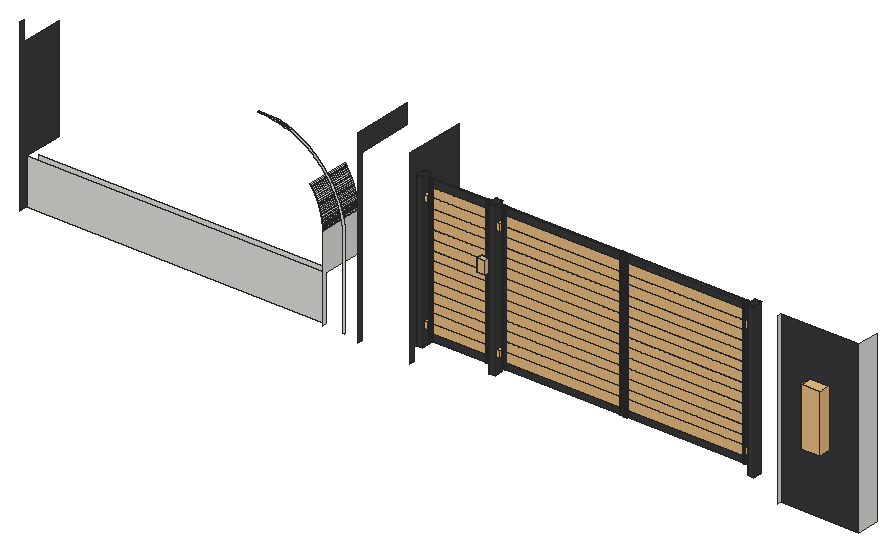
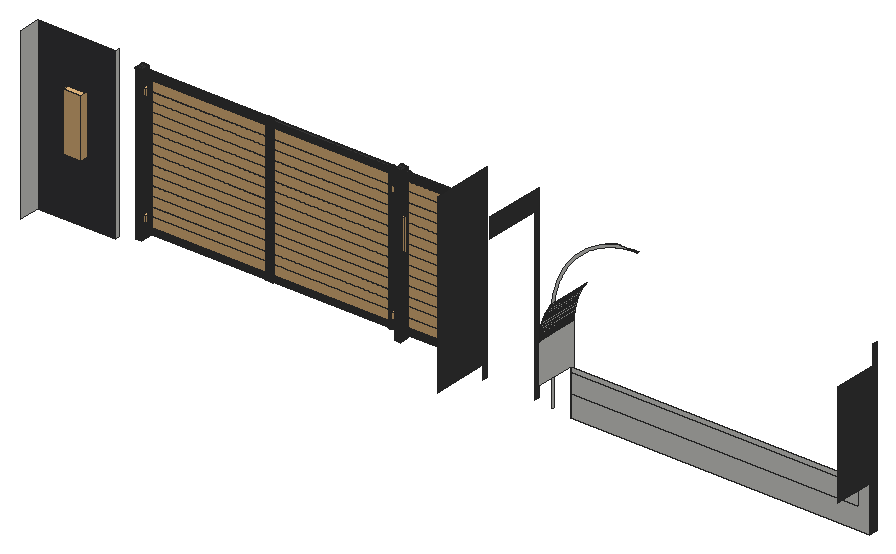
# SketchUp Ruby script. Lengths in inches.
U = 1.inch
M = Sketchup.active_model
def pt(a) = Geom::Point3d.new(a.map { |v| v * U })
def face(e, loops, mat)
  f = e.add_face(loops[0].map { |a| pt(a) })
  loops[1..].each { |l| e.add_face(l.map { |a| pt(a) }).erase! }
  f.material = f.back_material = mat if mat
  f
end
# faces: each face lists its corners as indices into pts; further lists are holes
def faces(e, pts, list, mat = nil) = list.each { |f| face(e, (f[0].is_a?(Array) ? f : [f]).map { |l| l.map { |i| pts[i] } }, mat) }
# xy, xz, yz: faces in a plane at the given z, y or x. An outline is a flat list of corners, or four numbers for a rectangle; further outlines are holes
def ring(l) = l.size == 4 ? [[l[0], l[1]], [l[2], l[1]], [l[2], l[3]], [l[0], l[3]]] : l.each_slice(2).to_a
def flat(e, list, mat, &to3) = list.each { |f| face(e, (f[0].is_a?(Array) ? f : [f]).map { |l| ring(l).map { |u, v| to3.(u, v) } }, mat) }
def xy(e, z, list, mat = nil) = flat(e, list, mat) { |x, y| [x, y, z] }
def xz(e, y, list, mat = nil) = flat(e, list, mat) { |x, z| [x, y, z] }
def yz(e, x, list, mat = nil) = flat(e, list, mat) { |y, z| [x, y, z] }
def lines(e, pts, list) = list.each { |a, b| e.add_line(pt(pts[a]), pt(pts[b])) }
# prism: a flat outline (further loops are holes) pulled along v
def prism(e, loops, v, mat = nil)
  f = face(e, loops, mat); d = Geom::Vector3d.new(v.map { |x| x * U })
  f.pushpull(f.normal.samedirection?(d) ? d.length : -d.length)
end
def box(e, o, s, mat = nil) = prism(e, [[o, [o[0] + s[0], o[1], o[2]], [o[0] + s[0], o[1] + s[1], o[2]], [o[0], o[1] + s[1], o[2]]]], [0, 0, s[2]], mat)
def at(x, y, z, deg = 0) = Geom::Transformation.translation(pt([x, y, z])) * Geom::Transformation.rotation(ORIGIN, Z_AXIS, deg.degrees)
def axes(o, x, y, z) = Geom::Transformation.new([*x, 0, *y, 0, *z, 0, *pt(o).to_a, 1])
def part(name) = M.definitions.add(name)
# library, detail: a bought-in or finely detailed component or shape, given as its bounding box
def library(name, o, s) = part(name).tap { |d| box(d.entities, o, s) }
def detail(e, o, s) = box(e.add_group.entities, o, s)
def put(e, d, t, mat = nil) = e.add_instance(d, t).tap { |i| i.material = mat if mat }
def group(e, t, mat = nil) = e.add_group.tap { |g| g.transformation = t; g.material = mat if mat }.entities
root = M.entities
M.materials.add("1432 AP 8245 TAR ROAD").color = [57, 57, 60]
M.materials.add("[Color M06]").color = [58, 58, 58]
M.materials.add("[Granite Dark Gray]").color = [61, 60, 60]
c1 = library("WALL LIGHT 61",[-1.86,-2.6875,-10.98],[8.43,8.43,26.69])
c2 = part("lamel up")
xy(c2.entities,0,[[[41.063,0.29,42.441,2.047],[41.122,0.389,42.343,1.973]],[[3.268,0.315,4.646,2.047],[3.327,0.389,4.587,1.973]]])
xy(c2.entities,4.331,[[3.327,0.439,4.587,1.924],[41.122,0.439,42.343,1.924]])
xy(c2.entities,4.724,[[4.646,0.439,41.063,1.924]])
xy(c2.entities,7.874,[[[3.268,0.315,4.646,0.315,4.646,0.439,41.063,0.439,41.063,0.315,42.441,0.315,42.441,2.047,41.063,2.047,41.063,1.924,4.646,1.924,4.646,2.047,3.268,2.047],[3.327,0.389,3.327,1.973,4.587,1.973,4.587,1.924,3.327,1.924,3.327,0.439,4.587,0.439,4.587,0.389],[41.122,0.389,41.122,0.439,42.343,0.439,42.343,1.924,41.122,1.924,41.122,1.973,42.343,1.973,42.343,0.389]]])
xz(c2.entities,0.315,[[3.268,0,4.646,7.874]])
xz(c2.entities,0.389,[[3.327,0,4.587,7.874],[41.122,0,42.343,7.874]])
xz(c2.entities,0.439,[[3.327,4.331,4.587,7.874],[41.122,4.331,42.343,7.874],[4.646,4.724,41.063,7.874]])
xz(c2.entities,1.924,[[3.327,4.331,4.587,7.874],[41.122,4.331,42.343,7.874],[4.646,4.724,41.063,7.874]])
xz(c2.entities,1.973,[[3.327,0,4.587,7.874],[41.122,0,42.343,7.874]])
xz(c2.entities,2.047,[[3.268,0,4.646,7.874],[41.063,0,42.441,7.874]])
yz(c2.entities,3.268,[[0.315,0,2.047,7.874]])
yz(c2.entities,3.327,[[0.389,0,1.973,0,1.973,7.874,1.924,7.874,1.924,4.331,0.439,4.331,0.439,7.874,0.389,7.874],[0.439,4.331,1.924,7.874]])
yz(c2.entities,4.587,[[0.389,0,0.389,7.874,0.439,7.874,0.439,4.331,0.394,0],[0.394,0,0.439,4.331,1.924,4.331,1.969,0],[1.969,0,1.924,4.331,1.924,7.874,1.973,7.874,1.973,0]])
yz(c2.entities,4.646,[[0.315,0,2.047,0,2.047,7.874,1.924,7.874,1.924,4.724,0.439,4.724,0.439,7.874,0.315,7.874]])
yz(c2.entities,41.063,[[0.29,0,0.315,7.874,0.439,7.874,0.439,4.724,1.924,4.724,1.924,7.874,2.047,7.874,2.047,0]])
yz(c2.entities,41.122,[[0.389,0,0.394,0,0.389,2.887,0.439,4.331,0.439,7.874,0.389,7.874],[0.394,0,1.969,0,1.973,2.943,1.924,4.331,0.439,4.331,0.389,2.887],[1.969,0,1.973,0,1.973,7.874,1.924,7.874,1.924,4.331,1.973,2.943]])
yz(c2.entities,42.343,[[0.389,0,0.389,7.874,0.439,7.874,0.439,4.331,1.924,4.331,1.924,7.874,1.973,7.874,1.973,0],[0.439,4.331,1.924,7.874]])
yz(c2.entities,42.441,[[0.29,0,2.047,0,2.047,7.874,0.315,7.874]])
p = [[42.441,0.29,0],[42.441,0.315,7.874],[41.063,0.315,7.874],[41.063,0.29,0]]
faces(c2.entities,p,[[0,1,2,3]])
c3 = library("lamel",[3.23,0.1,0.39],[36.57,1.38,4.33])
c4 = part("Gate stile")
xy(c4.entities,0,[[0.08,0.39,0.16,0.47],[0.16,0.39,0.16,0.47,1.57,0.47,1.57,0.59,1.65,0.59,1.65,0.39],[1.65,0.39,1.65,0.59,1.71,0.59,1.71,0.45,2.52,0.45,2.52,0.39],[0.08,0.47,0.08,1.97,1.65,1.97,1.65,1.77,1.57,1.77,1.57,1.89,0.16,1.89,0.16,0.47],[1.65,1.77,1.65,1.97,2.52,1.97,2.52,1.91,1.71,1.91,1.71,1.77]])
xy(c4.entities,3.15,[[1.57,0.59,1.65,1.77],[1.65,0.59,1.71,1.77]])
xy(c4.entities,63.78,[[1.57,0.59,1.65,1.77],[1.65,0.59,1.71,1.77]])
xy(c4.entities,66.93,[[0.08,0.39,1.65,0.39,1.65,0.59,1.57,0.59,1.57,0.47,0.16,0.47,0.16,1.89,1.57,1.89,1.57,1.77,1.65,1.77,1.65,1.97,0.08,1.97],[1.65,0.39,2.52,0.39,2.52,0.45,1.71,0.45,1.71,0.59,1.65,0.59],[1.65,1.77,1.71,1.77,1.71,1.91,2.52,1.91,2.52,1.97,1.65,1.97]])
xz(c4.entities,0.39,[[0.08,0,1.65,66.93],[1.65,0,2.52,66.93]])
xz(c4.entities,0.45,[[1.71,0,2.52,66.93]])
xz(c4.entities,0.47,[[0.16,0,1.57,66.93]])
xz(c4.entities,0.59,[[1.57,0,1.65,3.15],[1.65,0,1.71,3.15],[1.57,63.78,1.65,66.93],[1.65,63.78,1.71,66.93]])
xz(c4.entities,1.77,[[1.57,0,1.65,3.15],[1.65,0,1.71,3.15],[1.57,63.78,1.65,66.93],[1.65,63.78,1.71,66.93]])
xz(c4.entities,1.89,[[0.16,0,1.57,66.93]])
xz(c4.entities,1.91,[[1.71,0,2.52,66.93]])
xz(c4.entities,1.97,[[0.08,0,1.65,66.93],[1.65,0,2.52,66.93]])
yz(c4.entities,0.08,[[0.39,0,1.97,66.93]])
yz(c4.entities,0.16,[[0.47,0,1.89,66.93]])
yz(c4.entities,1.57,[[0.47,0,0.59,3.15],[1.77,0,1.89,3.15],[0.47,3.15,0.59,63.78],[0.59,3.15,0.59,63.78,1.77,3.15],[1.77,3.15,0.59,63.78,1.76,9.24],
  [1.77,3.15,1.76,9.24,1.89,3.15],[1.89,3.15,1.76,9.24,1.77,63.78,1.89,63.78],[1.76,9.24,0.59,63.78,1.77,63.78],[0.47,63.78,0.59,66.93],[1.77,63.78,1.89,66.93]])
yz(c4.entities,1.65,[[0.39,0,0.59,0,0.59,3.15,1.77,3.15,1.77,0,1.97,0,1.97,66.93,1.77,66.93,1.77,63.78,0.59,63.78,0.59,66.93,0.39,66.93]])
yz(c4.entities,1.71,[[0.45,0,0.59,0,0.59,3.15,1.77,3.15,1.77,0,1.91,0,1.91,63.78,0.45,63.78],[0.45,63.78,0.59,66.93],[1.77,63.78,1.91,66.93]])
yz(c4.entities,2.52,[[0.39,0,0.45,66.93],[1.91,0,1.97,66.93]])
c5 = part("Gate post")
xy(c5.entities,-3.9375,[[0.2,0.2,4.13,4.13]])
xy(c5.entities,66.93,[[[0,0,4.33,4.33],[0.2,0.2,4.13,4.13]]])
xy(c5.entities,67.01,[[0.2,0.2,4.13,4.13]])
xy(c5.entities,67.52,[[1.3,1.3,3.03,3.03]])
xz(c5.entities,0,[[0,66.93,4.33,67.01]])
xz(c5.entities,0.2,[[0.2,-3.9375,4.13,66.93],[0.2,66.93,4.13,67.01]])
xz(c5.entities,4.13,[[0.2,-3.9375,4.13,66.93],[0.2,66.93,4.13,67.01]])
xz(c5.entities,4.33,[[0,66.93,4.33,67.01]])
yz(c5.entities,0,[[0,66.93,4.33,67.01]])
yz(c5.entities,0.2,[[0.2,-3.9375,4.13,66.93],[0.2,66.93,4.13,67.01]])
yz(c5.entities,4.13,[[0.2,-3.9375,4.13,66.93],[0.2,66.93,4.13,67.01]])
yz(c5.entities,4.33,[[0,66.93,4.33,67.01]])
p = [[1.3,1.3,67.52],[1.3,3.03,67.52],[0,4.33,67.01],[0,0,67.01],[4.33,0,67.01],[3.03,1.3,67.52],
  [4.33,4.33,67.01],[3.03,3.03,67.52]]
faces(c5.entities,p,[[0,1,2,3],[4,5,0,3],[4,6,7,5],[2,1,7,6]])
c6 = library("skp6A9D",[-1.57,-1.57,-0.47],[3.14,3.14,2.95])
c7 = library("skp798A",[-3.31,-3.5,-20.01],[6.62,4.76,40.02])
c8 = library("Handle",[560.53,1368.21,-900.68],[5,2.66,5.75])
c9 = library("lamel\#1",[-36.14,0.1,0.39],[75.94,1.38,4.33])
c10 = part("lamel up\#1")
xy(c10.entities,0,[[[41.063,0.29,42.441,2.047],[41.122,0.389,42.343,1.973]],[[-36.102,0.315,-34.724,2.047],[-36.043,0.389,-34.783,1.973]]])
xy(c10.entities,4.331,[[-36.043,0.439,-34.783,1.924],[41.122,0.439,42.343,1.924]])
xy(c10.entities,4.724,[[-34.724,0.439,41.063,1.924]])
xy(c10.entities,7.874,[[[-36.102,0.315,-34.724,0.315,-34.724,0.439,41.063,0.439,41.063,0.315,42.441,0.315,42.441,2.047,41.063,2.047,41.063,1.924,-34.724,1.924,-34.724,2.047,-36.102,2.047],[-36.043,0.389,-36.043,1.973,-34.783,1.973,-34.783,1.924,-36.043,1.924,-36.043,0.439,-34.783,0.439,-34.783,0.389],[41.122,0.389,41.122,0.439,42.343,0.439,42.343,1.924,41.122,1.924,41.122,1.973,42.343,1.973,42.343,0.389]]])
xz(c10.entities,0.315,[[-36.102,0,-34.724,7.874]])
xz(c10.entities,0.389,[[-36.043,0,-34.783,7.874],[41.122,0,42.343,7.874]])
xz(c10.entities,0.439,[[-36.043,4.331,-34.783,7.874],[41.122,4.331,42.343,7.874],[-34.724,4.724,41.063,7.874]])
xz(c10.entities,1.924,[[-36.043,4.331,-34.783,7.874],[41.122,4.331,42.343,7.874],[-34.724,4.724,41.063,7.874]])
xz(c10.entities,1.973,[[-36.043,0,-34.783,7.874],[41.122,0,42.343,7.874]])
xz(c10.entities,2.047,[[-36.102,0,-34.724,7.874],[41.063,0,42.441,7.874]])
yz(c10.entities,-36.102,[[0.315,0,2.047,7.874]])
yz(c10.entities,-36.043,[[0.389,0,1.973,0,1.973,7.874,1.924,7.874,1.924,4.331,0.439,4.331,0.439,7.874,0.389,7.874],[0.439,4.331,1.924,7.874]])
yz(c10.entities,-34.783,[[0.389,0,0.389,7.874,0.439,7.874,0.439,4.331,0.394,0],[0.394,0,0.439,4.331,1.924,4.331,1.969,0],[1.969,0,1.924,4.331,1.924,7.874,1.973,7.874,1.973,0]])
yz(c10.entities,-34.724,[[0.315,0,2.047,0,2.047,7.874,1.924,7.874,1.924,4.724,0.439,4.724,0.439,7.874,0.315,7.874]])
yz(c10.entities,41.063,[[0.29,0,0.315,7.874,0.439,7.874,0.439,4.724,1.924,4.724,1.924,7.874,2.047,7.874,2.047,0]])
yz(c10.entities,41.122,[[0.389,0,0.394,0,0.389,2.887,0.439,4.331,0.439,7.874,0.389,7.874],[0.394,0,1.969,0,1.973,2.943,1.924,4.331,0.439,4.331,0.389,2.887],[1.969,0,1.973,0,1.973,7.874,1.924,7.874,1.924,4.331,1.973,2.943]])
yz(c10.entities,42.343,[[0.389,0,0.389,7.874,0.439,7.874,0.439,4.331,1.924,4.331,1.924,7.874,1.973,7.874,1.973,0],[0.439,4.331,1.924,7.874]])
yz(c10.entities,42.441,[[0.29,0,2.047,0,2.047,7.874,0.315,7.874]])
p = [[42.441,0.29,0],[42.441,0.315,7.874],[41.063,0.315,7.874],[41.063,0.29,0]]
faces(c10.entities,p,[[0,1,2,3]])
c11 = part("lamel up\#2")
xy(c11.entities,0,[[[41.063,0.29,42.441,2.047],[41.122,0.389,42.343,1.973]],[[-36.102,0.315,-34.724,2.047],[-36.043,0.389,-34.783,1.973]]])
xy(c11.entities,4.331,[[-36.043,0.439,-34.783,1.924],[41.122,0.439,42.343,1.924]])
xy(c11.entities,4.724,[[-34.724,0.439,41.063,1.924]])
xy(c11.entities,7.874,[[[-36.102,0.315,-34.724,0.315,-34.724,0.439,41.063,0.439,41.063,0.315,42.441,0.315,42.441,2.047,41.063,2.047,41.063,1.924,-34.724,1.924,-34.724,2.047,-36.102,2.047],[-36.043,0.389,-36.043,1.973,-34.783,1.973,-34.783,1.924,-36.043,1.924,-36.043,0.439,-34.783,0.439,-34.783,0.389],[41.122,0.389,41.122,0.439,42.343,0.439,42.343,1.924,41.122,1.924,41.122,1.973,42.343,1.973,42.343,0.389]]])
xz(c11.entities,0.315,[[-36.102,0,-34.724,7.874]])
xz(c11.entities,0.389,[[-36.043,0,-34.783,7.874],[41.122,0,42.343,7.874]])
xz(c11.entities,0.439,[[-36.043,4.331,-34.783,7.874],[41.122,4.331,42.343,7.874],[-34.724,4.724,41.063,7.874]])
xz(c11.entities,1.924,[[-36.043,4.331,-34.783,7.874],[41.122,4.331,42.343,7.874],[-34.724,4.724,41.063,7.874]])
xz(c11.entities,1.973,[[-36.043,0,-34.783,7.874],[41.122,0,42.343,7.874]])
xz(c11.entities,2.047,[[-36.102,0,-34.724,7.874],[41.063,0,42.441,7.874]])
yz(c11.entities,-36.102,[[0.315,0,2.047,7.874]])
yz(c11.entities,-36.043,[[0.389,0,1.973,0,1.973,7.874,1.924,7.874,1.924,4.331,0.439,4.331,0.439,7.874,0.389,7.874],[0.439,4.331,1.924,7.874]])
yz(c11.entities,-34.783,[[0.389,0,0.389,7.874,0.439,7.874,0.439,4.331,0.394,0],[0.394,0,0.439,4.331,1.924,4.331,1.969,0],[1.969,0,1.924,4.331,1.924,7.874,1.973,7.874,1.973,0]])
yz(c11.entities,-34.724,[[0.315,0,2.047,0,2.047,7.874,1.924,7.874,1.924,4.724,0.439,4.724,0.439,7.874,0.315,7.874]])
yz(c11.entities,41.063,[[0.29,0,0.315,7.874,0.439,7.874,0.439,4.724,1.924,4.724,1.924,7.874,2.047,7.874,2.047,0]])
yz(c11.entities,41.122,[[0.389,0,0.394,0,0.389,2.887,0.439,4.331,0.439,7.874,0.389,7.874],[0.394,0,1.969,0,1.973,2.943,1.924,4.331,0.439,4.331,0.389,2.887],[1.969,0,1.973,0,1.973,7.874,1.924,7.874,1.924,4.331,1.973,2.943]])
yz(c11.entities,42.343,[[0.389,0,0.389,7.874,0.439,7.874,0.439,4.331,1.924,4.331,1.924,7.874,1.973,7.874,1.973,0],[0.439,4.331,1.924,7.874]])
yz(c11.entities,42.441,[[0.29,0,2.047,0,2.047,7.874,0.315,7.874]])
p = [[42.441,0.29,0],[42.441,0.315,7.874],[41.063,0.315,7.874],[41.063,0.29,0]]
faces(c11.entities,p,[[0,1,2,3]])
c12 = part("170_fin_black_gate")
put(c12.entities,c2,axes([44.17,-0.15,7.875],[-1,0,0],[0,0.79545,0],[0,0,-1]),"[Color M06]")
put(c12.entities,c3,at(42.85,1.57,41.73,-180),"[Color M06]")
put(c12.entities,c3,at(42.85,1.57,28.74,-180),"[Color M06]")
put(c12.entities,c3,at(42.85,1.57,54.72,-180),"[Color M06]")
put(c12.entities,c3,at(42.85,1.57,37.4,-180),"[Color M06]")
put(c12.entities,c3,at(42.85,1.57,46.0625,-180),"[Color M06]")
put(c12.entities,c3,at(42.85,1.57,50.39,-180),"[Color M06]")
put(c12.entities,c3,at(42.85,1.57,20.08,-180),"[Color M06]")
put(c12.entities,c3,at(42.85,1.57,7.09,-180),"[Color M06]")
put(c12.entities,c4,at(1.56,-0.39,0),"[Color M06]")
put(c12.entities,c2,axes([44.17,1.73,59.06],[-1,0,0],[0,-0.79545,0],[0,0,1]),"[Color M06]")
put(c12.entities,c3,at(42.85,1.57,24.41,-180),"[Color M06]")
put(c12.entities,c3,at(42.85,1.57,33.07,-180),"[Color M06]")
put(c12.entities,c3,at(42.85,1.57,15.75,-180),"[Color M06]")
put(c12.entities,c3,at(42.85,1.57,11.42,-180),"[Color M06]")
put(c12.entities,c3,at(42.85,1.57,2.76,-180),"[Color M06]")
put(c12.entities,c4,at(41.08,1.97,0,-180),"[Color M06]")
put(c12.entities,c3,at(42.85,1.57,59.06,-180),"[Color M06]")
put(c12.entities,c5,at(41.94,-1.42,0.59),"[Color M06]")
put(c12.entities,c5,at(-4.89,-1.42,0.59),"[Color M06]")
put(c12.entities,c6,axes([-0.76,0.79,58.55],[0,0.9966,0],[0,0,0.9966],[0.9966,0,0]),"[Color M06]")
put(c12.entities,c6,axes([-0.76,0.79,6.11],[0,0.9966,0],[0,0,0.9966],[0.9966,0,0]),"[Color M06]")
put(c12.entities,c7,axes([41.58,1.03,41.4],[0,-0.3825,0],[0.4425,0,0],[0,0,0.36105]),"[Color M06]")
put(c12.entities,c8,axes([601.55,-1370.97,938.8125],[-1,0,0],[0,1,0],[0,0,1]),"[Color M06]")
put(c12.entities,c9,at(89.77,1.67,33.07,-180),"[Color M06]")
put(c12.entities,c10,axes([91.09,1.82,59.06],[-1,0,0],[0,-0.79545,0],[0,0,1]),"[Color M06]")
put(c12.entities,c9,at(89.77,1.67,37.4,-180),"[Color M06]")
put(c12.entities,c9,at(89.77,1.67,41.73,-180),"[Color M06]")
put(c12.entities,c9,at(89.77,1.67,59.06,-180),"[Color M06]")
put(c12.entities,c4,at(127.37,2.0625,0,-180),"[Color M06]")
put(c12.entities,c9,at(89.77,1.67,46.0625,-180),"[Color M06]")
put(c12.entities,c9,at(89.77,1.67,54.72,-180),"[Color M06]")
put(c12.entities,c9,at(89.77,1.67,50.39,-180),"[Color M06]")
put(c12.entities,c9,at(89.77,1.67,7.09,-180),"[Color M06]")
put(c12.entities,c9,at(89.77,1.67,11.42,-180),"[Color M06]")
put(c12.entities,c9,at(89.77,1.67,28.74,-180),"[Color M06]")
put(c12.entities,c11,axes([91.09,-0.06,7.875],[-1,0,0],[0,0.79545,0],[0,0,-1]),"[Color M06]")
put(c12.entities,c4,at(48.47,-0.3,0),"[Color M06]")
put(c12.entities,c9,at(89.77,1.67,15.75,-180),"[Color M06]")
put(c12.entities,c9,at(89.77,1.67,24.41,-180),"[Color M06]")
put(c12.entities,c9,at(89.77,1.67,2.76,-180),"[Color M06]")
put(c12.entities,c9,at(89.77,1.67,20.08,-180),"[Color M06]")
put(c12.entities,c9,at(168.98,1.67,15.75,-180),"[Color M06]")
put(c12.entities,c9,at(168.98,1.67,24.41,-180),"[Color M06]")
put(c12.entities,c9,at(168.98,1.67,50.39,-180),"[Color M06]")
put(c12.entities,c4,at(127.68,-0.3,0),"[Color M06]")
put(c12.entities,c9,at(168.98,1.67,46.0625,-180),"[Color M06]")
put(c12.entities,c11,axes([170.3,-0.06,7.875],[-1,0,0],[0,0.79545,0],[0,0,-1]),"[Color M06]")
put(c12.entities,c9,at(168.98,1.67,2.76,-180),"[Color M06]")
put(c12.entities,c9,at(168.98,1.67,54.72,-180),"[Color M06]")
put(c12.entities,c9,at(168.98,1.67,11.42,-180),"[Color M06]")
put(c12.entities,c9,at(168.98,1.67,7.09,-180),"[Color M06]")
put(c12.entities,c9,at(168.98,1.67,28.74,-180),"[Color M06]")
put(c12.entities,c9,at(168.98,1.67,20.08,-180),"[Color M06]")
put(c12.entities,c9,at(168.98,1.67,33.07,-180),"[Color M06]")
put(c12.entities,c10,axes([170.3,1.82,59.06],[-1,0,0],[0,-0.79545,0],[0,0,1]),"[Color M06]")
put(c12.entities,c9,at(168.98,1.67,41.73,-180),"[Color M06]")
put(c12.entities,c9,at(168.98,1.67,37.4,-180),"[Color M06]")
put(c12.entities,c4,at(206.58,2.0625,0,-180),"[Color M06]")
put(c12.entities,c9,at(168.98,1.67,59.06,-180),"[Color M06]")
put(c12.entities,c5,at(208.77,-1.32,0.59),"[Color M06]")
put(c12.entities,c6,axes([46.08,0.79,6.11],[0,0.9966,0],[0,0,0.9966],[0.9966,0,0]),"[Color M06]")
put(c12.entities,c6,axes([46.08,0.79,58.55],[0,0.9966,0],[0,0,0.9966],[0.9966,0,0]),"[Color M06]")
put(c12.entities,c6,axes([208.97,0.88,6.11],[0,-0.9966,0],[0,0,0.9966],[-0.9966,0,0]),"[Color M06]")
put(c12.entities,c6,axes([208.97,0.88,58.55],[0,-0.9966,0],[0,0,0.9966],[-0.9966,0,0]),"[Color M06]")
xy(root,66,[[120,60,120.51,60.5]])
xz(root,60.5,[[159,-12,160,-12,160,27.52,159.99,28.05,159.95,29.09,159.91,29.62,159.875,30.14,159.83,30.66,159.78,31.18,159.66,32.22,159.59,32.74,159.51,33.26,159.42,33.77,159.33,34.29,159.23,34.8,159.125,35.32,159.01,35.83,158.77,36.85,158.64,37.35,158.5,37.86,158.2,38.86,157.88,39.86,157.71,40.35,157.53,40.84,156.96,42.31,156.33,43.75,156.1,44.22,155.875,44.69,155.64,45.16,155.4,45.625,155.15,46.09,154.9,46.54,154.64,47,154.11,47.9,153.83,48.34,153.55,48.79,153.26,49.22,152.97,49.66,152.67,50.09,152.05,50.93,151.73,51.35,151.09,52.17,150.75,52.58,150.42,52.98,150.07,53.375,149.73,53.77,148.65,54.91,147.91,55.65,146.77,56.73,146.375,57.07,145.98,57.42,145.58,57.75,145.17,58.09,144.35,58.73,143.93,59.05,143.09,59.67,142.66,59.97,142.22,60.26,141.79,60.55,141.34,60.83,140.9,61.11,140,61.64,139.54,61.9,139.09,62.15,138.625,62.4,138.16,62.64,137.69,62.875,137.22,63.1,136.75,63.33,135.31,63.96,133.84,64.53,133.35,64.71,132.86,64.88,131.86,65.2,130.86,65.5,130.35,65.64,129.85,65.77,129.34,65.89,128.89,66,120,66,120.51,66,121.02,65.99,122.04,65.95,122.55,65.92,123.57,65.84,124.08,65.79,124.58,65.73,125.09,65.67,125.6,65.6,126.1,65.52,126.6,65.4375,127.11,65.35,128.11,65.15,128.61,65.04,129.1,64.92,129.6,64.8,130.09,64.67,130.59,64.54,131.08,64.39,131.57,64.25,132.05,64.09,132.54,63.93,133.5,63.59,133.98,63.41,134.92,63.03,135.4,62.83,135.86,62.63,136.33,62.42,137.25,61.98,137.71,61.75,139.06,61.03,139.5,60.77,139.94,60.52,140.38,60.25,140.8125,59.98,141.24,59.71,141.67,59.43,142.51,58.85,143.33,58.25,143.74,57.94,144.14,57.63,144.54,57.31,144.9375,56.98,145.33,56.66,145.71,56.32,146.1,55.98,146.47,55.64,146.85,55.29,147.21,54.9375,147.58,54.58,147.9375,54.21,148.29,53.85,148.64,53.47,148.98,53.1,149.32,52.71,149.66,52.33,149.98,51.9375,150.31,51.54,150.63,51.14,150.94,50.74,151.25,50.33,151.85,49.51,152.43,48.67,152.71,48.24,152.98,47.8125,153.25,47.38,153.52,46.94,153.77,46.5,154.03,46.06,154.75,44.71,154.98,44.25,155.42,43.33,155.63,42.86,155.83,42.4,156.03,41.92,156.41,40.98,156.59,40.5,156.93,39.54,157.09,39.05,157.25,38.57,157.39,38.08,157.54,37.59,157.67,37.09,157.8,36.6,157.92,36.1,158.04,35.61,158.15,35.11,158.35,34.11,158.4375,33.6,158.52,33.1,158.6,32.6,158.67,32.09,158.73,31.58,158.79,31.08,158.84,30.57,158.92,29.55,158.95,29.04,158.99,28.02,159,27.51]])
xz(root,62,[[12,-12,150,9]])
xz(root,62,[[360,-12,396,66]],"1432 AP 8245 TAR ROAD")
xz(root,65,[[15,0,147,9]])
yz(root,12,[[58,-12,62,-12,62,9,80,9,80,57,60,57,60,66,58,66]],"[Granite Dark Gray]")
yz(root,150,[[60,-12,60,27,80,27,80,9,62,9,62,-12],[60,27,80,27.39]])
yz(root,168,[[58,-12,58,75,86,75,86,66,60,66,60,-12]],"[Granite Dark Gray]")
yz(root,192,[[58,-12,60,-12,60,-6,86,-6,86,75,58,75]],"[Granite Dark Gray]")
yz(root,360,[[60,-12,62,66]])
yz(root,396,[[62,-12,72,66]])
p = [[150,80,27.39],[150,60,27.39],[149.99,60,27.79],[149.99,80,27.79],[149.98,60,28.18],[149.98,80,28.18],
  [149.96,60,28.57],[149.96,80,28.57],[149.9375,60,28.96],[149.9375,80,28.96],[149.91,60,29.35],[149.91,80,29.35],
  [149.875,60,29.75],[149.875,80,29.75],[149.84,60,30.14],[149.84,80,30.14],[149.79,60,30.53],[149.79,80,30.53],
  [149.74,60,30.92],[149.74,80,30.92],[149.69,60,31.3],[149.69,80,31.3],[149.63,60,31.69],[149.63,80,31.69],
  [149.57,60,32.08],[149.57,80,32.08],[149.5,60,32.47],[149.5,80,32.47],[149.42,60,32.85],[149.42,80,32.85],
  [149.34,60,33.24],[149.34,80,33.24],[149.26,60,33.62],[149.26,80,33.62],[149.17,60,34],[149.17,80,34],
  [149.08,60,34.38],[149.08,80,34.38],[148.98,60,34.76],[148.98,80,34.76],[148.875,60,35.14],[148.875,80,35.14],
  [148.76,60,35.52],[148.76,80,35.52],[148.65,60,35.9],[148.65,80,35.9],[148.53,60,36.27],[148.53,80,36.27],
  [148.41,60,36.64],[148.41,80,36.64],[148.28,60,37.01],[148.28,80,37.01],[148.15,60,37.38],[148.15,80,37.38],
  [148.01,60,37.75],[148.01,80,37.75],[147.86,60,38.12],[147.86,80,38.12],[147.72,60,38.48],[147.72,80,38.48],
  [147.5625,60,38.84],[147.5625,80,38.84],[147.41,60,39.2],[147.41,80,39.2],[147.24,60,39.56],[147.24,80,39.56],
  [147.08,60,39.92],[147.08,80,39.92],[146.91,60,40.27],[146.91,80,40.27],[146.73,60,40.62],[146.73,80,40.62],
  [146.55,60,40.97],[146.55,80,40.97],[146.36,60,41.31],[146.36,80,41.31],[146.17,60,41.66],[146.17,80,41.66],
  [145.98,60,42],[145.98,80,42],[145.78,60,42.34],[145.78,80,42.34],[145.58,60,42.67],[145.58,80,42.67],
  [145.37,60,43.01],[145.37,80,43.01],[145.16,60,43.34],[145.16,80,43.34],[144.94,60,43.67],[144.94,80,43.67],
  [144.72,60,43.99],[144.72,80,43.99],[144.5,60,44.3125],[144.5,80,44.3125],[144.27,60,44.63],[144.27,80,44.63],
  [132.54,60,63.93],[133.02,60,63.76],[133.02,60.5,63.76],[132.54,60.5,63.93],[132.05,60,64.09],[132.05,60.5,64.09],
  [135.31,60,63.96],[134.82,60,64.15],[134.82,60.5,64.15],[135.31,60.5,63.96],[131.57,60,64.25],[131.57,60.5,64.25],
  [131.08,60,64.39],[131.08,60.5,64.39],[134.33,60,64.34],[134.33,60.5,64.34],[133.84,60,64.53],[133.84,60.5,64.53],
  [130.59,60,64.54],[130.59,60.5,64.54],[130.09,60,64.67],[130.09,60.5,64.67],[133.35,60,64.71],[133.35,60.5,64.71],
  [129.6,60,64.8],[129.6,60.5,64.8],[132.86,60,64.88],[132.86,60.5,64.88],[129.1,60,64.92],[129.1,60.5,64.92],
  [128.61,60,65.04],[128.61,60.5,65.04],[132.36,60,65.04],[132.36,60.5,65.04],[128.11,60,65.15],[128.11,60.5,65.15],
  [131.86,60,65.2],[131.86,60.5,65.2],[127.61,60,65.25],[127.61,60.5,65.25],[131.36,60,65.35],[131.36,60.5,65.35],
  [126.6,60,65.4375],[127.11,60,65.35],[127.11,60.5,65.35],[126.6,60.5,65.4375],[126.1,60,65.52],[126.1,60.5,65.52],
  [130.86,60,65.5],[130.86,60.5,65.5],[125.6,60,65.6],[125.6,60.5,65.6],[130.35,60,65.64],[130.35,60.5,65.64],
  [125.09,60,65.67],[125.09,60.5,65.67],[129.85,60,65.77],[129.85,60.5,65.77],[124.08,60,65.79],[124.58,60,65.73],
  [124.58,60.5,65.73],[124.08,60.5,65.79],[123.06,60,65.88],[123.57,60,65.84],[123.57,60.5,65.84],[123.06,60.5,65.88],
  [129.34,60,65.89],[129.34,60.5,65.89],[121.53,60,65.97],[122.04,60,65.95],[122.04,60.5,65.95],[121.53,60.5,65.97],
  [122.55,60,65.92],[122.55,60.5,65.92],[128.89,60,66],[128.89,60.5,66],[120.51,60,66],[121.02,60,65.99],
  [121.02,60.5,65.99],[120.51,60.5,66],[159,62,27],[159,60.5,27],[160,62,27],[160,60.5,27]]
faces(root,p,[[0,1,2,3],[3,2,4,5],[5,4,6,7],[7,6,8,9],[9,8,10,11],[11,10,12,13],[13,12,14,15],[15,14,16,17],
  [17,16,18,19],[19,18,20,21],[21,20,22,23],[23,22,24,25],[25,24,26,27],[27,26,28,29],[29,28,30,31],[31,30,32,33],
  [33,32,34,35],[35,34,36,37],[37,36,38,39],[39,38,40,41],[41,40,42,43],[43,42,44,45],[45,44,46,47],[47,46,48,49],
  [49,48,50,51],[51,50,52,53],[53,52,54,55],[55,54,56,57],[57,56,58,59],[59,58,60,61],[61,60,62,63],[63,62,64,65],
  [65,64,66,67],[67,66,68,69],[69,68,70,71],[71,70,72,73],[73,72,74,75],[75,74,76,77],[77,76,78,79],[79,78,80,81],
  [81,80,82,83],[83,82,84,85],[85,84,86,87],[87,86,88,89],[89,88,90,91],[91,90,92,93],[93,92,94,95],[96,97,98,99],
  [100,96,99,101],[102,103,104,105],[106,100,101,107],[108,106,107,109],[103,110,111,104],[110,112,113,111],[114,108,109,115],[116,114,115,117],
  [112,118,119,113],[120,116,117,121],[118,122,123,119],[124,120,121,125],[126,124,125,127],[122,128,129,123],[130,126,127,131],[128,132,133,129],
  [134,130,131,135],[132,136,137,133],[138,139,140,141],[139,134,135,140],[142,138,141,143],[136,144,145,137],[146,142,143,147],[144,148,149,145],
  [150,146,147,151],[148,152,153,149],[154,155,156,157],[155,150,151,156],[158,159,160,161],[159,154,157,160],[152,162,163,153],[164,165,166,167],
  [165,168,169,166],[168,158,161,169],[162,170,171,163],[172,173,174,175],[173,164,167,174]])
lines(root,p,[[176,177],[178,179]])
put(root,c1,at(375.37,59.44,28.04))
put(root,c12,axes([195.5,62.76,-2.65],[0.71561,0,0],[0,1,0],[0,0,0.9996]))
